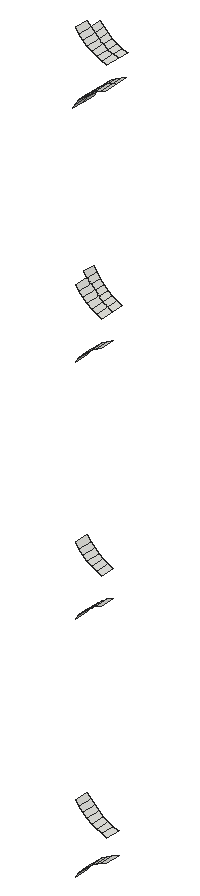
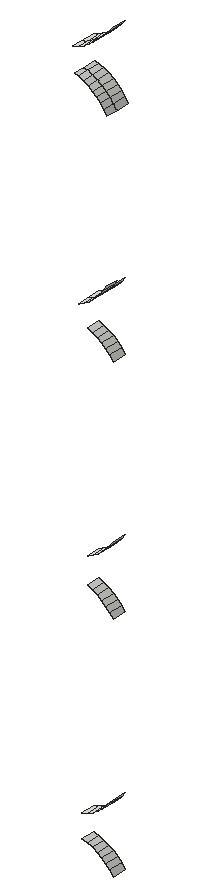
# SketchUp Ruby script. Lengths in inches.
U = 1.inch
M = Sketchup.active_model
def pt(a) = Geom::Point3d.new(a.map { |v| v * U })
def face(e, loops, mat)
  f = e.add_face(loops[0].map { |a| pt(a) })
  loops[1..].each { |l| e.add_face(l.map { |a| pt(a) }).erase! }
  f.material = f.back_material = mat if mat
  f
end
# faces: each face lists its corners as indices into pts; further lists are holes
def faces(e, pts, list, mat = nil) = list.each { |f| face(e, (f[0].is_a?(Array) ? f : [f]).map { |l| l.map { |i| pts[i] } }, mat) }
# xy, xz, yz: faces in a plane at the given z, y or x. An outline is a flat list of corners, or four numbers for a rectangle; further outlines are holes
def ring(l) = l.size == 4 ? [[l[0], l[1]], [l[2], l[1]], [l[2], l[3]], [l[0], l[3]]] : l.each_slice(2).to_a
def flat(e, list, mat, &to3) = list.each { |f| face(e, (f[0].is_a?(Array) ? f : [f]).map { |l| ring(l).map { |u, v| to3.(u, v) } }, mat) }
def xy(e, z, list, mat = nil) = flat(e, list, mat) { |x, y| [x, y, z] }
def xz(e, y, list, mat = nil) = flat(e, list, mat) { |x, z| [x, y, z] }
def yz(e, x, list, mat = nil) = flat(e, list, mat) { |y, z| [x, y, z] }
def lines(e, pts, list) = list.each { |a, b| e.add_line(pt(pts[a]), pt(pts[b])) }
# prism: a flat outline (further loops are holes) pulled along v
def prism(e, loops, v, mat = nil)
  f = face(e, loops, mat); d = Geom::Vector3d.new(v.map { |x| x * U })
  f.pushpull(f.normal.samedirection?(d) ? d.length : -d.length)
end
def box(e, o, s, mat = nil) = prism(e, [[o, [o[0] + s[0], o[1], o[2]], [o[0] + s[0], o[1] + s[1], o[2]], [o[0], o[1] + s[1], o[2]]]], [0, 0, s[2]], mat)
def at(x, y, z, deg = 0) = Geom::Transformation.translation(pt([x, y, z])) * Geom::Transformation.rotation(ORIGIN, Z_AXIS, deg.degrees)
def axes(o, x, y, z) = Geom::Transformation.new([*x, 0, *y, 0, *z, 0, *pt(o).to_a, 1])
def part(name) = M.definitions.add(name)
# library, detail: a bought-in or finely detailed component or shape, given as its bounding box
def library(name, o, s) = part(name).tap { |d| box(d.entities, o, s) }
def detail(e, o, s) = box(e.add_group.entities, o, s)
def put(e, d, t, mat = nil) = e.add_instance(d, t).tap { |i| i.material = mat if mat }
def group(e, t, mat = nil) = e.add_group.tap { |g| g.transformation = t; g.material = mat if mat }.entities
root = M.entities
p = [[79.8,138.79,8.56],[79.99,138.79,8.82],[79.99,138,8.82],[79.8,138,8.56],[80.21,138.79,9.05],[80.21,138,9.05],
  [80.44,138.79,9.26],[80.44,138,9.26],[80.7,138.79,9.45],[80.7,138,9.45],[80.97,138.79,9.62],[80.97,138,9.62],
  [81.26,138.79,9.75],[81.26,138,9.75],[81.56,138.79,9.86],[81.56,138,9.86],[81.56,138.79,11.14],[81.26,138.79,11.25],
  [81.26,138,11.25],[81.56,138,11.14],[80.97,138.79,11.38],[80.97,138,11.38],[80.7,138.79,11.55],[80.7,138,11.55],
  [80.44,138.79,11.74],[80.44,138,11.74],[80.21,138.79,11.95],[80.21,138,11.95],[79.99,138.79,12.18],[79.99,138,12.18],
  [79.8,138.79,12.44],[79.8,138,12.44],[79.8,138.79,21.56],[79.99,138.79,21.82],[79.99,138,21.82],[79.8,138,21.56],
  [80.21,138.79,22.05],[80.21,138,22.05],[80.44,138.79,22.26],[80.44,138,22.26],[80.7,138.79,22.45],[80.7,138,22.45],
  [80.97,138.79,22.62],[80.97,138,22.62],[81.26,138.79,22.75],[81.26,138,22.75],[81.26,138.79,24.25],[80.97,138.79,24.38],
  [80.97,138,24.38],[81.26,138,24.25],[80.7,138.79,24.55],[80.7,138,24.55],[80.44,138.79,24.74],[80.44,138,24.74],
  [80.21,138.79,24.95],[80.21,138,24.95],[79.99,138.79,25.18],[79.99,138,25.18],[79.8,138.79,25.44],[79.8,138,25.44],
  [79.8,138.79,34.56],[79.99,138.79,34.82],[79.99,138,34.82],[79.8,138,34.56],[80.21,138.79,35.05],[80.21,138,35.05],
  [80.44,138.79,35.26],[80.44,138,35.26],[80.7,138.79,35.45],[80.7,138,35.45],[80.97,138.79,35.62],[80.97,138,35.62],
  [81.26,138.79,35.75],[81.26,138,35.75],[81.26,138.79,37.25],[80.97,138.79,37.38],[80.97,138,37.38],[81.26,138,37.25],
  [80.97,139.4375,37.38],[81.26,139.4375,37.25],[80.7,138.79,37.55],[80.7,138,37.55],[80.7,139.4375,37.55],[80.44,138.79,37.74],
  [80.44,138,37.74],[80.44,139.4375,37.74],[80.21,138.79,37.95],[80.21,138,37.95],[80.21,139.4375,37.95],[79.99,138.79,38.18],
  [79.99,138,38.18],[79.99,139.4375,38.18],[79.8,138.79,38.44],[79.8,138,38.44],[79.8,139.4375,38.44],[79.64,139.4375,38.71],
  [79.64,138.79,38.71],[79.64,138.79,47.29],[79.8,138.79,47.56],[79.8,138,47.56],[79.64,138,47.29],[79.8,139.4375,47.56],
  [79.64,139.4375,47.29],[79.99,138.79,47.82],[79.99,138,47.82],[79.99,139.4375,47.82],[80.21,138.79,48.05],[80.21,138,48.05],
  [80.21,139.4375,48.05],[80.44,138.79,48.26],[80.44,138,48.26],[80.44,139.4375,48.26],[80.7,138.79,48.45],[80.7,138,48.45],
  [80.7,139.4375,48.45],[80.97,138.79,48.62],[80.97,138,48.62],[80.97,139.4375,48.62],[81.26,138.79,48.75],[81.26,138,48.75],
  [81.26,139.4375,48.75],[81.46,138.79,48.82],[81.46,138,48.82],[81.46,139.4375,48.82],[81.26,138,50.25],[81.56,138,50.14],
  [81.56,138.79,50.14],[81.26,138.79,50.25],[81.26,139.4375,50.25],[81.56,139.4375,50.14],[80.97,138.79,50.38],[80.97,138,50.38],
  [80.97,139.4375,50.38],[80.7,138.79,50.55],[80.7,138,50.55],[80.7,139.4375,50.55],[80.44,138.79,50.74],[80.44,138,50.74],
  [80.44,139.4375,50.74],[80.21,138.79,50.95],[80.21,138,50.95],[80.21,139.4375,50.95],[79.99,138.79,51.18],[79.99,138,51.18],
  [79.99,139.4375,51.18],[79.8,138.79,51.44],[79.8,138,51.44]]
faces(root,p,[[0,1,2,3],[1,4,5,2],[4,6,7,5],[6,8,9,7],[8,10,11,9],[10,12,13,11],[12,14,15,13],[16,17,18,19],
  [17,20,21,18],[20,22,23,21],[22,24,25,23],[24,26,27,25],[26,28,29,27],[28,30,31,29],[32,33,34,35],[33,36,37,34],
  [36,38,39,37],[38,40,41,39],[40,42,43,41],[42,44,45,43],[46,47,48,49],[47,50,51,48],[50,52,53,51],[52,54,55,53],
  [54,56,57,55],[56,58,59,57],[60,61,62,63],[61,64,65,62],[64,66,67,65],[66,68,69,67],[68,70,71,69],[70,72,73,71],
  [74,75,76,77],[78,75,74,79],[75,80,81,76],[82,80,75,78],[80,83,84,81],[85,83,80,82],[83,86,87,84],[88,86,83,85],
  [86,89,90,87],[91,89,86,88],[89,92,93,90],[94,92,89,91],[95,96,92,94],[97,98,99,100],[101,98,97,102],[98,103,104,99],
  [105,103,98,101],[103,106,107,104],[108,106,103,105],[106,109,110,107],[111,109,106,108],[109,112,113,110],[114,112,109,111],[112,115,116,113],
  [117,115,112,114],[115,118,119,116],[120,118,115,117],[118,121,122,119],[123,121,118,120],[124,125,126,127],[128,127,126,129],[127,130,131,124],
  [132,130,127,128],[130,133,134,131],[135,133,130,132],[133,136,137,134],[138,136,133,135],[136,139,140,137],[141,139,136,138],[139,142,143,140],
  [144,142,139,141],[142,145,146,143]])
